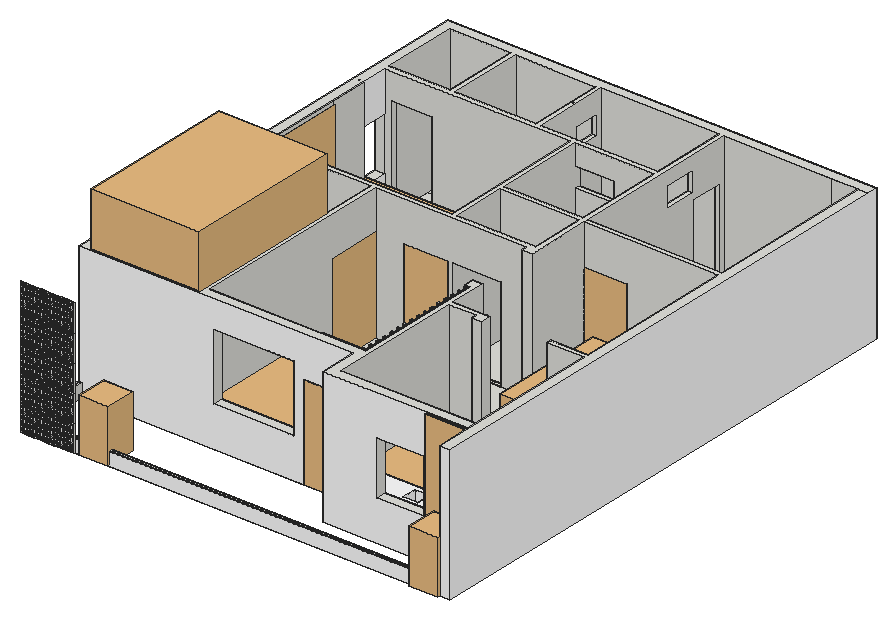
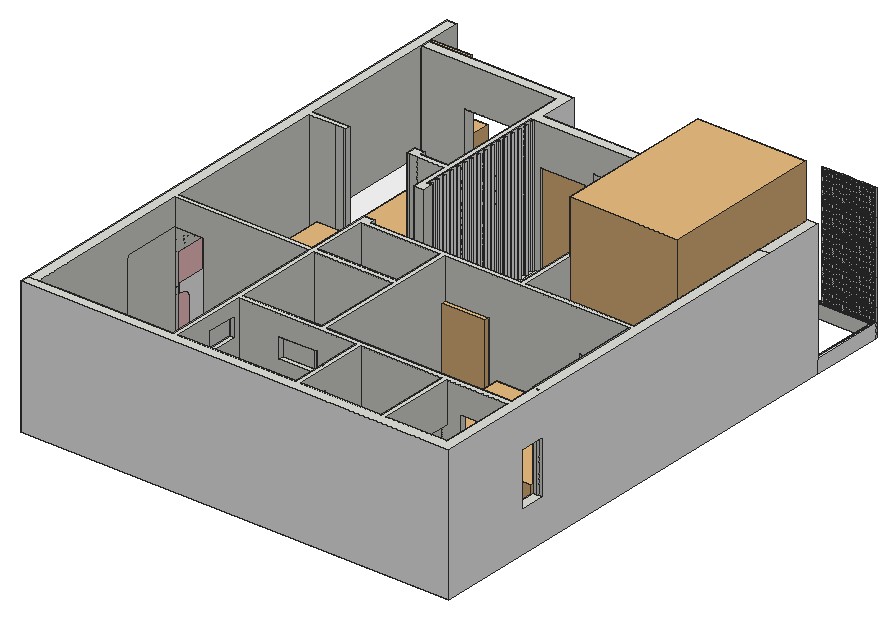
# SketchUp Ruby script. Lengths in inches.
U = 1.inch
M = Sketchup.active_model
def pt(a) = Geom::Point3d.new(a.map { |v| v * U })
def face(e, loops, mat)
  f = e.add_face(loops[0].map { |a| pt(a) })
  loops[1..].each { |l| e.add_face(l.map { |a| pt(a) }).erase! }
  f.material = f.back_material = mat if mat
  f
end
# faces: each face lists its corners as indices into pts; further lists are holes
def faces(e, pts, list, mat = nil) = list.each { |f| face(e, (f[0].is_a?(Array) ? f : [f]).map { |l| l.map { |i| pts[i] } }, mat) }
# xy, xz, yz: faces in a plane at the given z, y or x. An outline is a flat list of corners, or four numbers for a rectangle; further outlines are holes
def ring(l) = l.size == 4 ? [[l[0], l[1]], [l[2], l[1]], [l[2], l[3]], [l[0], l[3]]] : l.each_slice(2).to_a
def flat(e, list, mat, &to3) = list.each { |f| face(e, (f[0].is_a?(Array) ? f : [f]).map { |l| ring(l).map { |u, v| to3.(u, v) } }, mat) }
def xy(e, z, list, mat = nil) = flat(e, list, mat) { |x, y| [x, y, z] }
def xz(e, y, list, mat = nil) = flat(e, list, mat) { |x, z| [x, y, z] }
def yz(e, x, list, mat = nil) = flat(e, list, mat) { |y, z| [x, y, z] }
def lines(e, pts, list) = list.each { |a, b| e.add_line(pt(pts[a]), pt(pts[b])) }
# prism: a flat outline (further loops are holes) pulled along v
def prism(e, loops, v, mat = nil)
  f = face(e, loops, mat); d = Geom::Vector3d.new(v.map { |x| x * U })
  f.pushpull(f.normal.samedirection?(d) ? d.length : -d.length)
end
def box(e, o, s, mat = nil) = prism(e, [[o, [o[0] + s[0], o[1], o[2]], [o[0] + s[0], o[1] + s[1], o[2]], [o[0], o[1] + s[1], o[2]]]], [0, 0, s[2]], mat)
def at(x, y, z, deg = 0) = Geom::Transformation.translation(pt([x, y, z])) * Geom::Transformation.rotation(ORIGIN, Z_AXIS, deg.degrees)
def axes(o, x, y, z) = Geom::Transformation.new([*x, 0, *y, 0, *z, 0, *pt(o).to_a, 1])
def part(name) = M.definitions.add(name)
# library, detail: a bought-in or finely detailed component or shape, given as its bounding box
def library(name, o, s) = part(name).tap { |d| box(d.entities, o, s) }
def detail(e, o, s) = box(e.add_group.entities, o, s)
def put(e, d, t, mat = nil) = e.add_instance(d, t).tap { |i| i.material = mat if mat }
def group(e, t, mat = nil) = e.add_group.tap { |g| g.transformation = t; g.material = mat if mat }.entities
root = M.entities
M.materials.add("6755 marble 8.5cm").color = [255, 255, 255]
M.materials.add("Carpaint White 004 1.79cm\#5").color = [255, 255, 255]
M.materials.add("Ceramic Sand 8.13cm").color = [255, 255, 255]
M.materials.add("Manhattan Creative Coating MD 1125B 26.44cm").color = [255, 255, 255]
M.materials.add("Manhattan Creative Coating ML 1016B 24.75cm").color = [255, 255, 255]
M.materials.add("Wood 003 15.64cm").color = [255, 255, 255]
M.materials.add("Wood 021 27.52cm").color = [255, 255, 255]
M.materials.add("Wood Amboyan 13.2cm").color = [255, 255, 255]
M.materials.add("[Carrera Marble]").color = [207, 207, 207]
M.materials.add("[Color A01]").color = [255, 204, 204]
M.materials.add("[Wood Veneer 01]").color = [120, 70, 37]
c1 = part("Decorative lattice panel")
xy(c1.entities,0,[[0,-1,6,0]])
xy(c1.entities,0.42,[[0.75,-1,2.58,0]],"Wood 003 15.64cm")
xy(c1.entities,0.65,[[3.65,-1,4.84,0]],"Wood 003 15.64cm")
xy(c1.entities,23.35,[[0.65,-1,1.7,0],[4.3,-1,5.35,0]],"Wood 003 15.64cm")
xy(c1.entities,24,[[0,-1,6,0]])
xz(c1.entities,-1,[[[0,0,6,24],[5.58,11.5,3.49,14.96,5.58,18.43],[0.42,11.5,0.42,18.43,2.51,14.96],[2.58,6.51,0.49,9.97,2.58,13.44],[3.42,6.51,3.42,13.44,5.51,9.97],[5.58,1.52,3.49,4.99,5.58,8.45],[0.42,1.52,0.42,8.45,2.51,4.99],[2.58,16.48,0.51,19.93,2.58,22.72],[3.42,16.48,3.42,22.72,5.49,19.93],[0.75,0.42,2.58,3.47,2.58,0.42],[3.65,0.65,3.65,2.63,4.84,0.65],[0.65,21.93,0.65,23.35,1.7,23.35],[5.35,21.93,4.3,23.35,5.35,23.35]]],"Wood 003 15.64cm")
xz(c1.entities,0,[[[0,0,6,24],[5.58,11.5,5.58,18.43,3.49,14.96],[0.42,11.5,2.51,14.96,0.42,18.43],[2.58,6.51,2.58,13.44,0.49,9.97],[3.42,6.51,5.51,9.97,3.42,13.44],[5.58,1.52,5.58,8.45,3.49,4.99],[0.42,1.52,2.51,4.99,0.42,8.45],[2.58,16.48,2.58,22.72,0.51,19.93],[3.42,16.48,5.49,19.93,3.42,22.72],[0.75,0.42,2.58,0.42,2.58,3.47],[3.65,0.65,4.84,0.65,3.65,2.63],[0.65,21.93,1.7,23.35,0.65,23.35],[5.35,21.93,5.35,23.35,4.3,23.35]]])
yz(c1.entities,0,[[-1,0,0,24]])
yz(c1.entities,0.42,[[-1,1.52,0,8.45],[-1,11.5,0,18.43]],"Wood 003 15.64cm")
yz(c1.entities,0.65,[[-1,21.93,0,23.35]],"Wood 003 15.64cm")
yz(c1.entities,2.58,[[-1,0.42,0,3.47],[-1,6.51,0,13.44],[-1,16.48,0,22.72]],"Wood 003 15.64cm")
yz(c1.entities,3.42,[[-1,6.51,0,13.44],[-1,16.48,0,22.72]],"Wood 003 15.64cm")
yz(c1.entities,3.65,[[-1,0.65,0,2.63]],"Wood 003 15.64cm")
yz(c1.entities,5.35,[[-1,21.93,0,23.35]],"Wood 003 15.64cm")
yz(c1.entities,5.58,[[-1,1.52,0,8.45],[-1,11.5,0,18.43]],"Wood 003 15.64cm")
yz(c1.entities,6,[[-1,0,0,24]])
p = [[0.75,0,0.42],[2.58,0,3.47],[2.58,-1,3.47],[0.75,-1,0.42],[3.65,0,2.63],[4.84,0,0.65],
  [4.84,-1,0.65],[3.65,-1,2.63],[2.51,0,4.99],[0.42,0,1.52],[0.42,-1,1.52],[2.51,-1,4.99],
  [5.58,0,1.52],[3.49,0,4.99],[3.49,-1,4.99],[5.58,-1,1.52],[0.42,0,8.45],[0.42,-1,8.45],
  [5.58,0,8.45],[5.58,-1,8.45],[2.58,0,6.51],[0.49,0,9.97],[0.49,-1,9.97],[2.58,-1,6.51],
  [5.51,0,9.97],[3.42,0,6.51],[3.42,-1,6.51],[5.51,-1,9.97],[2.58,0,13.44],[2.58,-1,13.44],
  [3.42,0,13.44],[3.42,-1,13.44],[2.51,0,14.96],[0.42,0,11.5],[0.42,-1,11.5],[2.51,-1,14.96],
  [5.58,0,11.5],[3.49,0,14.96],[3.49,-1,14.96],[5.58,-1,11.5],[0.42,0,18.43],[0.42,-1,18.43],
  [5.58,0,18.43],[5.58,-1,18.43],[2.58,0,16.48],[0.51,0,19.93],[0.51,-1,19.93],[2.58,-1,16.48],
  [5.49,0,19.93],[3.42,0,16.48],[3.42,-1,16.48],[5.49,-1,19.93],[2.58,0,22.72],[2.58,-1,22.72],
  [3.42,0,22.72],[3.42,-1,22.72],[1.7,0,23.35],[0.65,0,21.93],[0.65,-1,21.93],[1.7,-1,23.35],
  [5.35,0,21.93],[4.3,0,23.35],[4.3,-1,23.35],[5.35,-1,21.93]]
faces(c1.entities,p,[[0,1,2,3],[4,5,6,7],[8,9,10,11],[12,13,14,15],[16,8,11,17],[13,18,19,14],[20,21,22,23],[24,25,26,27],
  [21,28,29,22],[30,24,27,31],[32,33,34,35],[36,37,38,39],[40,32,35,41],[37,42,43,38],[44,45,46,47],[48,49,50,51],
  [45,52,53,46],[54,48,51,55],[56,57,58,59],[60,61,62,63]],"Wood 003 15.64cm")
c2 = part("Group\#140")
put(c2.entities,c1,at(18,0,0))
put(c2.entities,c1,at(12,0,0))
put(c2.entities,c1,at(6,0,0))
put(c2.entities,c1,at(0,0,0))
put(c2.entities,c1,at(18,0,24))
put(c2.entities,c1,at(6,0,24))
put(c2.entities,c1,at(0,0,24))
put(c2.entities,c1,at(12,0,24))
put(c2.entities,c1,at(18,0,48))
put(c2.entities,c1,at(6,0,48))
put(c2.entities,c1,at(0,0,48))
put(c2.entities,c1,at(12,0,48))
put(c2.entities,c1,at(18,0,72))
put(c2.entities,c1,at(6,0,72))
put(c2.entities,c1,at(0,0,72))
put(c2.entities,c1,at(12,0,72))
put(c2.entities,c1,at(18,0,96))
put(c2.entities,c1,at(6,0,96))
put(c2.entities,c1,at(0,0,96))
put(c2.entities,c1,at(12,0,96))
c3 = library("Indoor Plant 010",[-15.15,-14.1,0],[25.78,27.29,47.64])
c4 = library("Group1493\#1",[-18,-60,0],[36,120,2])
c5 = part("OuterShell")
prism(c5.entities,[[[0,0,0.08],[0,0,0.31],[0,0.59,0.31],[0,0.59,0.39],[0,0.79,0.39],[0,0.79,0],[0,0.59,0],[0,0.59,0.08]]],[0.39,0,0])
c6 = part("Cabinet pull")
put(c6.entities,c5,at(0,0,0))
put(c6.entities,c5,at(8.62,0,0))
g1 = group(c6.entities,at(0,0,0))
g2 = group(g1,at(0,0,0.2))
xy(g2,0,[[0.39,0.39,8.62,0.79]])
xy(g2,0.12,[[0.39,0.39,8.62,0.59]])
xy(g2,0.2,[[0.39,0.59,8.62,0.63],[0.39,0.63,8.62,0.79]])
xz(g2,0.39,[[0.39,0,8.62,0.12]])
xz(g2,0.59,[[0.39,0.12,8.62,0.2]])
xz(g2,0.79,[[0.39,0,8.62,0.2]])
yz(g2,0.39,[[0.39,0,0.39,0.12,0.59,0.12,0.59,0.2,0.79,0.2,0.79,0]])
yz(g2,8.62,[[0.39,0,0.79,0,0.79,0.2,0.59,0.2,0.59,0.12,0.39,0.12]])
g3 = group(g1,at(0,0,0.2))
xy(g3,-0.2,[[0.39,0.59,8.62,0.63],[0.39,0.63,8.62,0.79]])
xy(g3,-0.12,[[0.39,0.39,8.62,0.59]])
xy(g3,0,[[0.39,0.39,8.62,0.79]])
xz(g3,0.39,[[0.39,-0.12,8.62,0]])
xz(g3,0.59,[[0.39,-0.2,8.62,-0.12]])
xz(g3,0.79,[[0.39,-0.2,8.62,0]])
yz(g3,0.39,[[0.59,-0.2,0.79,-0.2,0.79,0,0.39,0,0.39,-0.12,0.59,-0.12]])
yz(g3,8.62,[[0.59,-0.2,0.59,-0.12,0.39,-0.12,0.39,0,0.79,0,0.79,-0.2]])
c7 = library("ประตู",[99.61,0,0],[47.24,8.5625,80.71])
c8 = library("Group\#6",[-95,0,0],[96,96,30.0625])
c9 = part("Square post")
box(c9.entities,[-2,0,0],[2,2,120],"Wood 021 27.52cm")
c10 = library("Archie Sectional",[-59.99,-44.69,0],[94.95,99.96,31.82])
c11 = library("Group\#154",[0,0,0],[96.64,142.7,167.57])
c12 = library("Group\#59",[0,0,0],[24.1,13.79,48.57])
c13 = library("Dining Table",[-4.14,-4.14,0],[95.74,137.21,49.0625])
c14 = library("modern double door",[0,0,0],[3.2,48,90])
c15 = library("Group\#22",[0,0,0],[2.375,72.75,120])
c16 = library("Untitled (14)",[0,0,0],[7.13,36,83])
c17 = library("Double bed ensemble",[6.09,0.88,0],[81.44,100.66,42.94])
xy(root,126,[[373,193.88,409,194.96],[45,425.96,46,532.9],[385,478.46,387,529.99],[387,478.46,409,529.99]])
xy(root,129,[[384,478.46,385,504.15]],"[Color A01]")
xy(root,246,[[373,193.88,409,194.96],[45,425.96,46,532.9]])
xz(root,193.88,[[373,126,409,246]],"Wood Amboyan 13.2cm")
xz(root,425.96,[[45,126,46,246]])
xz(root,478.46,[[387,126,409,126,409,222,385,222,385,129,387,129]])
xz(root,478.46,[[384,129,385,222]],"[Color A01]")
xz(root,504.15,[[384,129,385,136.71]],"[Color A01]")
xz(root,532.9,[[45,126,46,246]])
yz(root,45,[[425.96,126,532.9,246]])
yz(root,46,[[426.96,126,434.12,126,434.12,141.39,434.125,141.77,434.13,142.16,434.14,142.54,434.18,143.32,434.2,143.7,434.22,144.09,434.25,144.47,434.28,144.86,434.31,145.24,434.34,145.625,434.38,146.01,434.42,146.39,434.47,146.78,434.57,147.54,434.625,147.92,434.68,148.31,434.74,148.6875,434.8,149.07,435.01,150.21,435.09,150.58,435.33,151.72,435.42,152.09,435.51,152.47,435.61,152.84,435.7,153.22,435.8,153.59,435.91,153.96,436.01,154.33,436.23,155.07,436.35,155.4375,436.47,155.81,436.59,156.17,436.71,156.54,436.84,156.9,436.97,157.27,437.23,157.99,437.51,158.71,437.81,159.43,437.96,159.78,438.11,160.14,438.26,160.49,438.58,161.19,438.75,161.54,438.91,161.89,439.08,162.24,439.26,162.58,439.43,162.92,439.61,163.27,439.97,163.95,440.16,164.29,440.35,164.62,440.54,164.96,440.74,165.29,440.93,165.62,441.33,166.28,441.54,166.61,441.75,166.93,441.96,167.26,442.17,167.58,442.39,167.9,442.6,168.22,442.82,168.54,443.05,168.85,443.27,169.16,443.73,169.78,443.97,170.09,444.2,170.4,444.4375,170.7,444.68,171,444.92,171.3,445.42,171.9,446.17,172.77,446.43,173.0625,446.69,173.35,446.95,173.63,447.22,173.91,447.48,174.19,447.75,174.47,448.02,174.74,448.29,175.02,448.85,175.56,449.125,175.82,449.41,176.09,449.69,176.35,449.98,176.61,450.27,176.86,450.56,177.12,451.14,177.62,451.4375,177.87,451.74,178.11,452.04,178.36,452.34,178.6,452.64,178.83,452.95,179.07,453.26,179.3,453.56,179.53,453.875,179.76,454.1875,179.99,454.5,180.21,455.14,180.65,455.46,180.86,455.78,181.08,456.11,181.29,456.43,181.49,456.76,181.7,457.75,182.3,458.08,182.49,458.42,182.68,458.76,182.875,459.09,183.06,459.77,183.42,460.12,183.6,460.46,183.78,460.81,183.95,461.15,184.12,461.5,184.28,461.85,184.45,462.55,184.77,462.91,184.92,463.26,185.08,463.62,185.23,463.97,185.375,464.33,185.52,464.69,185.66,465.16,185.84,466.08,186.22,467.46,186.82,467.92,187.03,468.37,187.24,469.27,187.68,469.72,187.91,470.16,188.13,470.61,188.37,471.05,188.6,471.49,188.85,471.92,189.09,472.36,189.34,472.79,189.59,473.65,190.11,474.49,190.64,474.91,190.92,475.33,191.19,475.75,191.47,476.57,192.05,476.97,192.34,477.38,192.63,478.18,193.23,478.58,193.54,479.36,194.16,479.75,194.48,480.13,194.8,480.89,195.45,481.27,195.78,481.64,196.12,482.01,196.45,482.38,196.79,483.46,197.84,484.17,198.55,484.51,198.91,484.86,199.27,485.54,200.01,485.87,200.38,486.53,201.14,487.17,201.9,487.49,202.29,487.8,202.68,488.11,203.08,488.42,203.47,489.02,204.27,489.3125,204.68,489.61,205.08,489.89,205.49,490.18,205.91,490.46,206.32,490.73,206.74,491.01,207.16,491.27,207.58,491.54,208.01,491.8,208.43,492.06,208.86,492.3125,209.3,492.56,209.73,492.8,210.17,493.05,210.61,493.28,211.05,493.52,211.49,493.75,211.94,493.97,212.38,494.41,213.28,494.62,213.74,494.83,214.19,495.43,215.57,495.62,216.03,495.81,216.5,495.99,216.96,496.35,217.9,496.52,218.37,496.68,218.84,496.84,219.32,497,219.79,497.3,220.75,497.45,221.22,497.59,221.71,497.72,222.1875,497.86,222.67,497.98,223.16,498.1,223.64,498.34,224.62,498.45,225.1,498.65,226.08,498.75,226.58,498.84,227.07,498.92,227.5625,499.01,228.05,499.08,228.55,499.16,229.04,499.22,229.54,499.29,230.04,499.35,230.53,499.5,232.03,499.58,233.03,499.64,234.03,499.68,235.03,499.71,236.53,499.71,237.03,499.7,237.53,499.7,238.03,499.64,239.53,499.55,241.03,499.51,241.53,499.36,243.03,499.3,243.52,499.23,244.02,499.17,244.52,499.09,245.01,499.02,245.51,498.93,246,426.96,246],[434.12,126,532.9,126,532.9,246,498.93,246,499.02,245.51,499.09,245.01,499.17,244.52,499.23,244.02,499.3,243.52,499.36,243.03,499.51,241.53,499.55,241.03,499.64,239.53,499.7,238.03,499.7,237.53,499.71,237.03,499.71,236.53,499.68,235.03,499.64,234.03,499.58,233.03,499.5,232.03,499.35,230.53,499.29,230.04,499.22,229.54,499.16,229.04,499.08,228.55,499.01,228.05,498.92,227.5625,498.84,227.07,498.75,226.58,498.65,226.08,498.45,225.1,498.34,224.62,498.1,223.64,497.98,223.16,497.86,222.67,497.72,222.1875,497.59,221.71,497.45,221.22,497.3,220.75,497,219.79,496.84,219.32,496.68,218.84,496.52,218.37,496.35,217.9,495.99,216.96,495.81,216.5,495.62,216.03,495.43,215.57,494.83,214.19,494.62,213.74,494.41,213.28,493.97,212.38,493.75,211.94,493.52,211.49,493.28,211.05,493.05,210.61,492.8,210.17,492.56,209.73,492.3125,209.3,492.06,208.86,491.8,208.43,491.54,208.01,491.27,207.58,491.01,207.16,490.73,206.74,490.46,206.32,490.18,205.91,489.89,205.49,489.61,205.08,489.3125,204.68,489.02,204.27,488.42,203.47,488.11,203.08,487.8,202.68,487.49,202.29,487.17,201.9,486.53,201.14,485.87,200.38,485.54,200.01,484.86,199.27,484.51,198.91,484.17,198.55,483.46,197.84,482.38,196.79,482.01,196.45,481.64,196.12,481.27,195.78,480.89,195.45,480.13,194.8,479.75,194.48,479.36,194.16,478.58,193.54,478.18,193.23,477.38,192.63,476.97,192.34,476.57,192.05,475.75,191.47,475.33,191.19,474.91,190.92,474.49,190.64,473.65,190.11,472.79,189.59,472.36,189.34,471.92,189.09,471.49,188.85,471.05,188.6,470.61,188.37,470.16,188.13,469.72,187.91,469.27,187.68,468.37,187.24,467.92,187.03,467.46,186.82,466.08,186.22,465.16,185.84,464.69,185.66,464.33,185.52,463.97,185.375,463.62,185.23,463.26,185.08,462.91,184.92,462.55,184.77,461.85,184.45,461.5,184.28,461.15,184.12,460.81,183.95,460.46,183.78,460.12,183.6,459.77,183.42,459.09,183.06,458.76,182.875,458.42,182.68,458.08,182.49,457.75,182.3,456.76,181.7,456.43,181.49,456.11,181.29,455.78,181.08,455.46,180.86,455.14,180.65,454.5,180.21,454.1875,179.99,453.875,179.76,453.56,179.53,453.26,179.3,452.95,179.07,452.64,178.83,452.34,178.6,452.04,178.36,451.74,178.11,451.4375,177.87,451.14,177.62,450.56,177.12,450.27,176.86,449.98,176.61,449.69,176.35,449.41,176.09,449.125,175.82,448.85,175.56,448.29,175.02,448.02,174.74,447.75,174.47,447.48,174.19,447.22,173.91,446.95,173.63,446.69,173.35,446.43,173.0625,446.17,172.77,445.42,171.9,444.92,171.3,444.68,171,444.4375,170.7,444.2,170.4,443.97,170.09,443.73,169.78,443.27,169.16,443.05,168.85,442.82,168.54,442.6,168.22,442.39,167.9,442.17,167.58,441.96,167.26,441.75,166.93,441.54,166.61,441.33,166.28,440.93,165.62,440.74,165.29,440.54,164.96,440.35,164.62,440.16,164.29,439.97,163.95,439.61,163.27,439.43,162.92,439.26,162.58,439.08,162.24,438.91,161.89,438.75,161.54,438.58,161.19,438.26,160.49,438.11,160.14,437.96,159.78,437.81,159.43,437.51,158.71,437.23,157.99,436.97,157.27,436.84,156.9,436.71,156.54,436.59,156.17,436.47,155.81,436.35,155.4375,436.23,155.07,436.01,154.33,435.91,153.96,435.8,153.59,435.7,153.22,435.61,152.84,435.51,152.47,435.42,152.09,435.33,151.72,435.09,150.58,435.01,150.21,434.8,149.07,434.74,148.6875,434.68,148.31,434.625,147.92,434.57,147.54,434.47,146.78,434.42,146.39,434.38,146.01,434.34,145.625,434.31,145.24,434.28,144.86,434.25,144.47,434.22,144.09,434.2,143.7,434.18,143.32,434.14,142.54,434.13,142.16,434.125,141.77,434.12,141.39]])
yz(root,373,[[193.88,126,194.96,246]],"Wood Amboyan 13.2cm")
yz(root,384,[[478.62,129,478.62,197.84,504.15,197.84,504.15,189.31,501.36,189.31,501.23,189.3,501.05,189.29,500.86,189.27,500.5,189.25,500.3125,189.24,500.21,189.23,500.13,189.22,499.77,189.14,499.58,189.1,499.4,189.07,499.22,189.03,499.07,189,499.03,188.99,498.85,188.92,498.67,188.86,498.49,188.79,498.3,188.73,498.12,188.67,497.98,188.62,497.9375,188.6,497.76,188.5,497.57,188.41,497.21,188.23,497.02,188.14,496.95,188.09,496.84,188.02,496.66,187.9,496.48,187.77,496.29,187.65,496.11,187.52,495.99,187.4375,495.93,187.39,495.75,187.22,495.5625,187.06,495.38,186.89,495.2,186.73,495.12,186.66,495.01,186.54,494.83,186.32,494.65,186.11,494.47,185.89,494.36,185.77,494.28,185.65,493.92,185.09,493.74,184.8125,493.72,184.78,493.55,184.44,493.37,184.0625,493.2,183.72,493.1875,183.67,493,183.11,492.83,182.6,492.82,182.54,492.64,181.59,492.61,181.44,492.53,180.25,492.53,145.77,492.61,144.58,492.64,144.43,492.82,143.48,492.83,143.42,493,142.91,493.1875,142.35,493.2,142.3,493.37,141.96,493.55,141.58,493.72,141.24,493.74,141.21,494.28,140.37,494.36,140.25,494.47,140.125,494.65,139.91,494.83,139.7,495.01,139.48,495.12,139.36,495.2,139.29,495.38,139.125,495.5625,138.96,495.75,138.8,495.93,138.63,495.99,138.58,496.11,138.5,496.29,138.37,496.48,138.25,496.84,137.99,496.95,137.92,497.02,137.88,497.21,137.79,497.57,137.61,497.76,137.51,497.9375,137.42,497.98,137.4,498.12,137.35,498.3,137.29,498.49,137.22,498.85,137.1,499.03,137.03,499.07,137.02,499.22,136.99,499.4,136.95,499.58,136.92,499.77,136.88,500.13,136.8,500.21,136.79,500.3125,136.78,500.5,136.77,500.68,136.76,500.86,136.74,501.05,136.73,501.23,136.72,501.36,136.71,504.15,136.71,504.15,129]],"Carpaint White 004 1.79cm\#5")
yz(root,384,[[478.46,129,478.62,222]],"[Color A01]")
yz(root,385,[[478.46,129,478.46,222,504.15,222,504.15,198,478.62,198,478.62,197.84,504.15,197.84,504.15,129]],"[Color A01]")
yz(root,387,[[478.46,126,529.99,129]],"[Wood Veneer 01]")
yz(root,409,[[193.88,126,194.96,246],[478.46,126,529.99,222]])
g4 = group(root,at(36,162.71,126))
put(g4,c2,at(0,1,0))
put(g4,c2,at(24,1,0))
put(root,c3,at(398.81,175.55,126))
put(root,c3,at(103.26,177.3,126))
put(root,c4,axes([391,193.88,186],[1,0,0],[0,0,1],[0,-1,0]),"Wood Amboyan 13.2cm")
g5 = group(root,at(36,163.71,126))
xy(g5,0,[[0,0,373,3],[0,3,3,64.25]])
xy(g5,12,[[0,0,373,0,373,1.5,1.5,1.5,1.5,64.25,0,64.25],[1.5,1.5,373,1.5,373,3,3,3,3,64.25,1.5,64.25]])
xz(g5,0,[[0,0,373,12]],"Manhattan Creative Coating MD 1125B 26.44cm")
xz(g5,3,[[3,0,373,12]])
xz(g5,64.25,[[0,0,3,12]])
yz(g5,0,[[0,0,64.25,12]],"Manhattan Creative Coating MD 1125B 26.44cm")
yz(g5,3,[[3,0,64.25,12]])
yz(g5,373,[[0,0,3,12]])
put(root,c6,axes([333.67,228.96,133.45],[1.23,0,0],[0,1,0],[0,0,1.36]))
put(root,c7,axes([154.28,227.96,126],[0.8255,0,0],[0,1,0],[0,0,1.04]))
g6 = group(root,at(289,203.96,126),"Wood 021 27.52cm")
xy(g6,0,[[[0,0,0,21,99,21,99,120,120,120,120,0],[49.9,6.43,63.18,19.375]]],"Wood 021 27.52cm")
xy(g6,3.9375,[[0,21,96,24],[96,21,99,120]],"Wood 021 27.52cm")
xy(g6,34,[[[0,0,120,0,120,120,96,120,96,24,0,24],[49.9,6.43,63.18,19.375]]],"Wood 021 27.52cm")
xz(g6,0,[[0,0,120,34]],"Wood 021 27.52cm")
xz(g6,6.43,[[49.9,0,63.18,34]],"Wood 021 27.52cm")
xz(g6,19.375,[[49.9,0,63.18,34]],"Wood 021 27.52cm")
xz(g6,21,[[0,0,99,3.9375]],"[Carrera Marble]")
xz(g6,24,[[0,3.9375,96,34]],"Wood 021 27.52cm")
xz(g6,120,[[99,0,99,3.9375,96,3.9375,96,34,120,34,120,0]],"Wood 021 27.52cm")
yz(g6,0,[[0,0,0,34,24,34,24,3.9375,21,3.9375,21,0]],"Wood 021 27.52cm")
yz(g6,49.9,[[6.43,0,19.375,34]],"Wood 021 27.52cm")
yz(g6,63.18,[[6.43,0,19.375,34]],"Wood 021 27.52cm")
yz(g6,96,[[24,3.9375,120,34]],"Wood 021 27.52cm")
yz(g6,99,[[21,0,120,3.9375]],"[Carrera Marble]")
yz(g6,120,[[0,0,120,34]],"Wood 021 27.52cm")
put(root,c8,at(384,227.96,129.9375),"Manhattan Creative Coating ML 1016B 24.75cm")
g7 = group(root,at(283.5,236.96,126),"Wood 021 27.52cm")
xy(g7,0,[[0,0,1,115.5]],"Wood 021 27.52cm")
xy(g7,120,[[0,0,1,115.5]],"Wood 021 27.52cm")
xz(g7,0,[[0,0,1,120]],"Wood 021 27.52cm")
xz(g7,115.5,[[0,0,1,120]],"Wood 021 27.52cm")
yz(g7,0,[[2,0,115.5,120]],"Wood 021 27.52cm")
yz(g7,1,[[0,0,115.5,120]],"Wood 021 27.52cm")
put(g7,c9,at(0,0,0))
put(g7,c9,at(0,7.57,0))
put(g7,c9,at(0,15.13,0))
put(g7,c9,at(0,22.7,0))
put(g7,c9,at(0,30.27,0))
put(g7,c9,at(0,37.83,0))
put(g7,c9,at(0,45.4,0))
put(g7,c9,at(0,52.97,0))
put(g7,c9,at(0,60.53,0))
put(g7,c9,at(0,68.1,0))
put(g7,c9,at(0,75.67,0))
put(g7,c9,at(0,83.23,0))
put(g7,c9,at(0,90.8,0))
put(g7,c9,at(0,98.37,0))
put(g7,c9,at(0,105.93,0))
put(g7,c9,at(0,113.5,0))
put(root,c10,axes([194.84,315.3,126],[0,1.30594,0],[-0.8928,0,0],[0,0,1]))
put(root,c11,at(45,229.96,126))
put(root,c12,at(80.57,363.92,126))
put(root,c13,axes([320.23,348.18,126],[0.75,0,0],[0,0.76,0],[0,0,1]))
put(root,c14,axes([145.75,421.46,126],[-1,0,0],[0,-1,0],[0,0,0.94]))
g8 = group(root,at(32.09,56.96,126))
xy(g8,0,[[376.91,106.75,376.91,417,295.91,417,295.91,421.5,376.91,421.5,376.91,573,385.91,573,385.91,106.75],[247.91,138,295.91,138,295.91,147,256.91,147,256.91,304.5,247.91,304.5,247.91,295.5,252.41,295.5,252.41,180,247.91,180],[256.91,147,376.91,147,376.91,267,343.91,267,343.91,262.5,352.91,262.5,352.91,171,256.91,171],[12.91,171,204.41,171,204.41,180,113.41,180,113.41,292,108.91,292,108.91,173,12.91,173],[243.41,171,247.91,180],
  [256.91,171,352.91,171,352.91,262.5,280.91,262.5,280.91,267,256.91,267],[113.41,180,116.41,180,116.41,301,142.48,301,142.48,304,113.41,304],[202.48,180,247.91,180,247.91,212.89,247.73,212.89,247.73,258.51,247.91,258.51,247.91,364.5,177.91,364.5,177.91,369,138.91,369,138.91,364.5,113.41,364.5,113.41,304,142.48,304,142.48,301,139.48,301,139.48,203,199.48,203,199.48,206,202.48,206],[247.91,180,252.41,180,252.41,295.5,247.91,295.5,247.91,258.51,250.55,258.51,250.55,212.89,247.91,212.89],[247.73,212.89,247.91,258.51],
  [247.91,212.89,250.55,258.51],[289.91,262.5,316.91,267,289.91,271.5],[289.91,262.5,343.91,262.5,316.91,267],[343.91,262.5,343.91,271.5,316.91,267],[316.91,267,343.91,271.5,289.91,271.5],
  [256.91,271.5,286.91,286.5],[286.91,271.5,346.91,271.5,346.91,286.5,376.91,286.5,376.91,320.25,367.91,320.25,367.91,368.25,376.91,368.25,376.91,417,295.91,417,295.91,421.5,256.91,421.5,256.91,286.5,286.91,286.5],[346.91,271.5,376.91,286.5],[247.91,304.5,252.41,332.25,247.91,360],[247.91,304.5,256.91,304.5,252.41,332.25],
  [256.91,304.5,256.91,360,252.41,332.25],[367.91,320.25,376.91,368.25],[252.41,332.25,256.91,360,247.91,360],[[247.91,360,256.91,360,256.91,510,252.41,510,252.41,505.5,177.91,505.5,177.91,364.5,182.41,364.5,182.41,421.5,212.41,421.5,212.41,417,252.41,417,252.41,369,225.41,369,225.41,364.5,247.91,364.5],[182.41,459,252.41,501]],[57.91,364.5,138.91,369],
  [182.41,364.5,203.91,366.75,182.41,369],[182.41,364.5,225.41,364.5,203.91,366.75],[225.41,364.5,225.41,369,203.91,366.75],[203.91,366.75,225.41,369,182.41,369],[12.91,369,177.91,501],
  [182.41,369,228.41,369,228.41,417,212.41,417,212.41,421.5,182.41,421.5],[228.41,369,252.41,417],[182.41,421.5,252.41,459],[256.91,421.5,352.91,421.5,352.91,472.125,364.91,472.125,364.91,520.125,352.91,520.125,352.91,573,256.91,573,256.91,568.5,252.41,568.5,252.41,538.5,256.91,538.5],[352.91,421.5,376.91,472.125],
  [182.41,459,252.41,501],[364.91,472.125,376.91,520.125],[3.91,501,3.91,582,385.91,582,385.91,573,147.91,573,147.91,568.5,143.41,568.5,143.41,573,71.41,573,71.41,535.5,66.91,535.5,66.91,573,12.91,573,12.91,501],[18.91,501,36.91,503.25,18.91,505.5],[18.91,501,54.91,501,36.91,503.25],
  [54.91,501,54.91,505.5,36.91,503.25],[54.91,501,147.91,501,147.91,544.5,143.41,544.5,143.41,505.5,54.91,505.5],[36.91,503.25,54.91,505.5,18.91,505.5],[12.91,505.5,71.41,505.5,71.41,535.5,66.91,535.5,66.91,549,12.91,549],[71.41,505.5,143.41,573],
  [147.91,505.5,252.41,573],[352.91,520.125,376.91,573],[12.91,549,66.91,573],[252.41,568.5,256.91,573]])
xy(g8,36,[[295.91,138,337.91,147],[123.91,171,195.91,180],[21.91,364.5,57.91,369],[3.91,477,12.91,501]])
xy(g8,84,[[295.91,138,337.91,147],[204.41,171,243.41,180],[108.91,316.5,113.41,364.5],[21.91,364.5,57.91,369],[138.91,364.5,177.91,369],
  [182.41,364.5,225.41,369],[182.41,417,212.41,421.5],[256.91,417,295.91,421.5],[3.91,477,12.91,501],[182.41,501,216.41,505.5],
  [66.91,505.5,71.41,535.5],[252.41,538.5,256.91,568.5],[143.41,544.5,147.91,568.5]])
xy(g8,90,[[252.41,510,256.91,538.5]])
xy(g8,96,[[123.91,171,195.91,180],[18.91,501,54.91,505.5]])
xy(g8,102,[[182.41,501,216.41,505.5],[143.41,544.5,147.91,568.5]])
xy(g8,108,[[252.41,510,256.91,538.5]])
xy(g8,120,[[376.91,106.75,385.91,106.75,385.91,573,376.91,573,376.91,421.5,256.91,421.5,256.91,417,376.91,417,376.91,271.5,343.91,271.5,343.91,267,376.91,267],[[247.91,138,376.91,138,376.91,147,256.91,147,256.91,267,280.91,267,280.91,262.5,289.91,262.5,289.91,271.5,256.91,271.5,256.91,304.5,247.91,304.5,247.91,295.5,252.41,295.5,252.41,180,113.41,180,113.41,364.5,247.91,364.5,247.91,360,256.91,360,256.91,573,385.91,573,385.91,582,3.91,582,3.91,224.62,12.91,226.58,12.91,364.5,57.91,364.5,57.91,369,12.91,369,12.91,501,177.91,501,177.91,369,57.91,369,57.91,364.5,108.91,364.5,108.91,173,12.91,173,12.91,171,247.91,171],[182.41,421.5,182.41,501,252.41,501,252.41,505.5,147.91,505.5,147.91,573,252.41,573,252.41,421.5],[71.41,505.5,143.41,573],[12.91,505.5,66.91,573],[182.41,369,252.41,417]],[3.91,171,12.91,171,12.91,226.58,3.91,224.62]])
xz(g8,106.75,[[376.91,0,385.91,120]],"Ceramic Sand 8.13cm")
xz(g8,138,[[247.91,0,337.91,0,337.91,36,295.91,36,295.91,84,337.91,84,337.91,0,376.91,0,376.91,120,247.91,120]],"Ceramic Sand 8.13cm")
xz(g8,147,[[[256.91,0,376.91,120],[295.91,36,337.91,84]]])
xz(g8,171,[[[3.91,0,204.41,0,204.41,84,243.41,84,243.41,0,247.91,0,247.91,120,3.91,120],[123.91,36,195.91,96]]],"Ceramic Sand 8.13cm")
xz(g8,173,[[12.91,0,108.91,120]])
xz(g8,180,[[[113.41,0,113.41,120,252.41,120,252.41,0,243.41,0,243.41,84,204.41,84,204.41,0],[123.91,36,195.91,96]]])
xz(g8,262.5,[[280.91,0,289.91,120]])
xz(g8,267,[[256.91,0,280.91,120],[343.91,0,376.91,120]])
xz(g8,271.5,[[256.91,0,280.91,120],[280.91,0,286.91,120],[286.91,0,289.91,120],[343.91,0,346.91,120],[346.91,0,352.91,120],
  [352.91,0,376.91,120]])
xz(g8,295.5,[[247.91,0,252.41,120]])
xz(g8,304.5,[[247.91,0,256.91,120]])
xz(g8,316.5,[[108.91,0,113.41,84]])
xz(g8,360,[[247.91,0,256.91,120]])
xz(g8,364.5,[[[12.91,0,138.91,0,138.91,84,177.91,84,177.91,0,182.41,0,182.41,84,225.41,84,225.41,0,247.91,0,247.91,120,113.41,120,113.41,84,108.91,84,108.91,120,12.91,120],[21.91,36,57.91,84]]])
xz(g8,369,[[[12.91,0,12.91,120,177.91,120,177.91,84,138.91,84,138.91,0],[21.91,36,57.91,84]],[225.41,0,225.41,84,182.41,84,182.41,120,252.41,120,252.41,0]])
xz(g8,417,[[212.41,0,252.41,0,252.41,120,182.41,120,182.41,84,212.41,84],[295.91,0,376.91,0,376.91,120,256.91,120,256.91,84,295.91,84]])
xz(g8,421.5,[[212.41,0,212.41,84,182.41,84,182.41,120,252.41,120,252.41,0],[295.91,0,295.91,84,256.91,84,256.91,120,376.91,120,376.91,0]])
xz(g8,477,[[3.91,36,7.61,84],[7.61,36,9.21,84],[9.21,36,12.91,84],[7.61,84,9.21,120]])
xz(g8,501,[[12.91,0,18.91,0,18.91,96,54.91,96,54.91,0,177.91,0,177.91,120,12.91,120],[182.41,0,216.41,84],[216.41,0,252.41,0,252.41,120,182.41,120,182.41,102,216.41,102],[3.91,36,12.91,84]])
xz(g8,505.5,[[12.91,0,12.91,120,66.91,120,66.91,84,71.41,84,71.41,0,54.91,0,54.91,96,18.91,96,18.91,0],[71.41,0,143.41,120],[147.91,0,147.91,120,252.41,120,252.41,0,182.41,0,182.41,84,216.41,84,216.41,102,182.41,102,182.41,0]])
xz(g8,510,[[252.41,90,256.91,108]])
xz(g8,535.5,[[66.91,0,71.41,84]])
xz(g8,538.5,[[252.41,0,256.91,84],[252.41,90,256.91,108]])
xz(g8,544.5,[[145.11,0,146.21,84],[143.41,84,145.11,102],[145.11,84,146.21,102],[146.21,84,147.91,102],[145.11,102,146.21,120]])
xz(g8,568.5,[[252.41,0,256.91,84],[143.41,84,147.91,102]])
xz(g8,573,[[12.91,0,66.91,120],[71.41,0,143.41,120],[147.91,0,252.41,120],[256.91,0,352.91,120],[352.91,0,376.91,120]])
xz(g8,582,[[3.91,0,385.91,120]],"Ceramic Sand 8.13cm")
yz(g8,3.91,[[[171,0,582,120],[477,36,501,84]]],"Ceramic Sand 8.13cm")
yz(g8,12.91,[[173,0,364.5,120],[505.5,0,573,120]])
yz(g8,12.91,[[369,0,501,0,501,36,477,36,477,84,501,84,501,120,369,120]],"6755 marble 8.5cm")
yz(g8,18.91,[[501,0,505.5,96]])
yz(g8,21.91,[[364.5,36,369,84]])
yz(g8,54.91,[[501,0,505.5,96]])
yz(g8,57.91,[[364.5,36,369,84]])
yz(g8,66.91,[[535.5,0,535.5,84,505.5,84,505.5,120,573,120,573,0]])
yz(g8,71.41,[[535.5,0,573,0,573,120,505.5,120,505.5,84,535.5,84]])
yz(g8,108.91,[[173,0,173,120,364.5,120,364.5,84,316.5,84,316.5,0]])
yz(g8,113.41,[[180,0,316.5,0,316.5,84,364.5,84,364.5,120,180,120]])
yz(g8,123.91,[[171,36,180,96]])
yz(g8,138.91,[[364.5,0,369,84]])
yz(g8,143.41,[[505.5,0,505.5,120,573,120,573,0,568.5,0,568.5,102,544.5,102,544.5,84,568.5,84,568.5,0]])
yz(g8,147.91,[[[505.5,0,573,120],[544.5,84,568.5,102]]])
yz(g8,177.91,[[364.5,0,369,84],[369,0,501,120]])
yz(g8,182.41,[[364.5,0,501,0,501,84,505.5,84,505.5,102,501,102,501,120,421.5,120,421.5,84,417,84,417,120,369,120,369,84,364.5,84]])
yz(g8,195.91,[[171,36,180,96]])
yz(g8,204.41,[[171,0,180,84]])
yz(g8,212.41,[[417,0,421.5,84]])
yz(g8,216.41,[[501,84,505.5,102]])
yz(g8,225.41,[[364.5,0,369,84]])
yz(g8,243.41,[[171,0,180,84]])
yz(g8,247.91,[[295.5,0,304.5,120],[360,0,364.5,120]])
yz(g8,247.91,[[138,0,171,120]],"Ceramic Sand 8.13cm")
yz(g8,252.41,[[180,0,295.5,120],[369,0,417,120],[421.5,0,501,120],[[505.5,0,505.5,120,573,120,573,0,568.5,0,568.5,84,538.5,84,538.5,0],[510,90,538.5,108]]])
yz(g8,256.91,[[147,0,267,120],[271.5,0,304.5,120],[360,0,421.5,0,421.5,84,417,84,417,120,360,120],[[421.5,0,538.5,0,538.5,84,568.5,84,568.5,0,573,0,573,120,421.5,120],[510,90,538.5,108]]])
yz(g8,280.91,[[262.5,0,267,120]])
yz(g8,289.91,[[262.5,0,271.5,120]])
yz(g8,295.91,[[417,0,421.5,84],[138,36,147,84]])
yz(g8,337.91,[[138,36,147,84]])
yz(g8,343.91,[[267,0,271.5,120]])
yz(g8,376.91,[[106.75,0,138,120],[138,0,147,120],[147,0,267,120],[271.5,0,417,120],[421.5,0,573,120]])
yz(g8,385.91,[[106.75,0,582,120]],"Ceramic Sand 8.13cm")
p = [[173.375,149.57,0],[173.6,149.26,0],[178.97,167.78,0],[178.81,167.43,0],[181.35,170.23,0],[181.02,170.03,0],
  [183.15,170.89,0],[182.77,170.8,0],[183.53,170.95,0],[183.91,170.99,0],[184.29,171,0],[69.91,312,0],
  [69.91,312.0625,0],[197.48,182,0],[163.48,182,0],[139.48,227,0],[118.41,227,0],[199.48,180,0],
  [199.48,203,0],[139.48,182,0],[139.48,203,0],[118.41,299,0],[139.48,299,0],[163.48,203,0],
  [139.48,275,0],[118.41,275,0],[118.41,182,0],[118.41,203,0],[139.48,251,0],[118.41,251,0],
  [197.48,203,0],[57.08,236.17,0],[57.82,236.34,0]]
lines(g8,p,[[0,1],[2,3],[4,5],[6,7],[8,6],[9,8],[10,9],[11,12],[13,14],[15,16],[17,18],[19,20],
  [21,22],[14,23],[24,25],[26,27],[28,29],[13,30],[25,21],[20,27],[19,26],[27,16],[14,19],[31,32],
  [29,25],[16,29]])
put(root,c7,axes([88.78,421.46,126],[0.8255,0,0],[0,1,0],[0,0,1.04]))
put(root,c15,axes([45,425.96,126],[1,0,0],[0,1,0],[0,0,0.98]),"Wood 021 27.52cm")
put(root,c16,axes([289,481.78,126],[0,-1,0],[1.08333,0,0],[0,0,1.01]))
put(root,c16,axes([214.5,483.34,126],[0,-1,0],[0.83333,0,0],[0,0,1.01]))
put(root,c17,axes([36.65,434.37,126],[1.37,0,0],[0,1,0],[0,0,1]))
